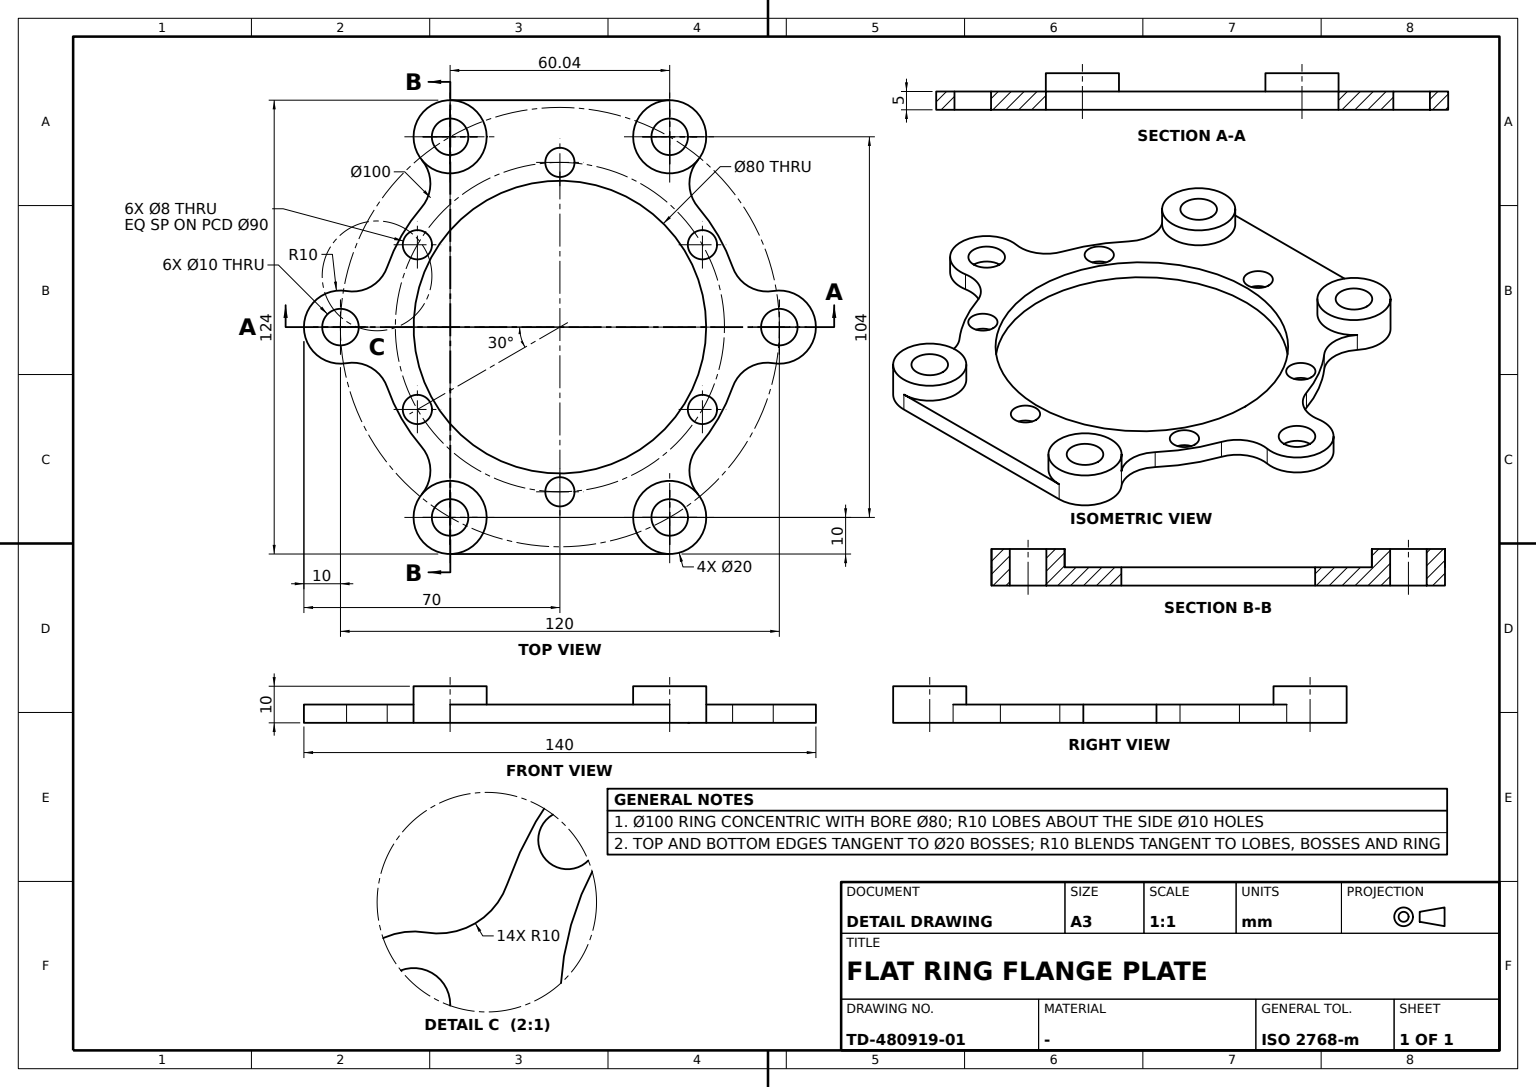
ISO-10303-21;
HEADER;
FILE_DESCRIPTION((''),'2;1');
FILE_NAME('','',(''),(''),'','','');
FILE_SCHEMA(('AUTOMOTIVE_DESIGN'));
ENDSEC;
DATA;
#1=APPLICATION_CONTEXT('');
#2=PRODUCT_CONTEXT('',#1,'mechanical');
#3=PRODUCT('','','',(#2));
#4=PRODUCT_DEFINITION_FORMATION('','',#3);
#5=PRODUCT_DEFINITION_CONTEXT('',#1,'design');
#6=PRODUCT_DEFINITION('','',#4,#5);
#7=PRODUCT_DEFINITION_SHAPE('','',#6);
#8=(LENGTH_UNIT()NAMED_UNIT(*)SI_UNIT(.MILLI.,.METRE.));
#9=(NAMED_UNIT(*)PLANE_ANGLE_UNIT()SI_UNIT($,.RADIAN.));
#10=(NAMED_UNIT(*)SI_UNIT($,.STERADIAN.)SOLID_ANGLE_UNIT());
#11=UNCERTAINTY_MEASURE_WITH_UNIT(LENGTH_MEASURE(0.005),#8,'distance_accuracy_value','');
#12=(GEOMETRIC_REPRESENTATION_CONTEXT(3)GLOBAL_UNCERTAINTY_ASSIGNED_CONTEXT((#11))GLOBAL_UNIT_ASSIGNED_CONTEXT((#8,#9,#10))REPRESENTATION_CONTEXT('',''));
#13=CARTESIAN_POINT('',(-37.8388717769,32.6836317237,0.));
#14=VERTEX_POINT('',#13);
#15=CARTESIAN_POINT('',(-37.7144300651,45.6101790342,0.));
#16=VERTEX_POINT('',#15);
#17=CARTESIAN_POINT('',(-45.4066461323,39.2203580684,0.));
#18=DIRECTION('',(0.,0.,1.));
#19=DIRECTION('',(1.,0.,0.));
#20=AXIS2_PLACEMENT_3D('',#17,#18,#19);
#21=CIRCLE('',#20,10.);
#22=EDGE_CURVE('',#14,#16,#21,.T.);
#23=ORIENTED_EDGE('',*,*,#22,.T.);
#24=CARTESIAN_POINT('',(-37.7144300651,45.6101790342,-5.));
#25=VERTEX_POINT('',#24);
#26=CARTESIAN_POINT('',(-37.7144300651,45.6101790342,-2.5));
#27=VECTOR('',#18,1000.);
#28=LINE('',#26,#27);
#29=EDGE_CURVE('',#16,#25,#28,.F.);
#30=ORIENTED_EDGE('',*,*,#29,.T.);
#31=CARTESIAN_POINT('',(-37.8388717769,32.6836317237,-5.));
#32=VERTEX_POINT('',#31);
#33=CARTESIAN_POINT('',(-45.4066461323,39.2203580684,-5.));
#34=AXIS2_PLACEMENT_3D('',#33,#18,#19);
#35=CIRCLE('',#34,10.);
#36=EDGE_CURVE('',#32,#25,#35,.T.);
#37=ORIENTED_EDGE('',*,*,#36,.F.);
#38=CARTESIAN_POINT('',(-37.8388717769,32.6836317237,-2.5));
#39=LINE('',#38,#27);
#40=EDGE_CURVE('',#14,#32,#39,.F.);
#41=ORIENTED_EDGE('',*,*,#40,.F.);
#42=EDGE_LOOP('',(#23,#30,#37,#41));
#43=FACE_BOUND('',#42,.T.);
#44=CARTESIAN_POINT('',(-45.4066461323,39.2203580684,-2.5));
#45=AXIS2_PLACEMENT_3D('',#44,#18,#19);
#46=CYLINDRICAL_SURFACE('',#45,10.);
#47=ADVANCED_FACE('',(#43),#46,.F.);
#48=CARTESIAN_POINT('',(-20.0222139979,52.,5.));
#49=VERTEX_POINT('',#48);
#50=CARTESIAN_POINT('',(-30.0222139979,52.,5.));
#51=AXIS2_PLACEMENT_3D('',#50,#18,#19);
#52=CIRCLE('',#51,10.);
#53=EDGE_CURVE('',#49,#49,#52,.T.);
#54=ORIENTED_EDGE('',*,*,#53,.T.);
#55=EDGE_LOOP('',(#54));
#56=FACE_BOUND('',#55,.T.);
#57=CARTESIAN_POINT('',(-25.0222139979,52.,5.));
#58=VERTEX_POINT('',#57);
#59=CIRCLE('',#51,5.);
#60=EDGE_CURVE('',#58,#58,#59,.T.);
#61=ORIENTED_EDGE('',*,*,#60,.F.);
#62=EDGE_LOOP('',(#61));
#63=FACE_BOUND('',#62,.T.);
#64=CARTESIAN_POINT('',(0.,0.,5.));
#65=AXIS2_PLACEMENT_3D('',#64,#18,#19);
#66=PLANE('',#65);
#67=ADVANCED_FACE('',(#56,#63),#66,.T.);
#68=CARTESIAN_POINT('',(-34.9711431703,-22.5,0.));
#69=VERTEX_POINT('',#68);
#70=CARTESIAN_POINT('',(-38.9711431703,-22.5,0.));
#71=AXIS2_PLACEMENT_3D('',#70,#18,#19);
#72=CIRCLE('',#71,4.);
#73=EDGE_CURVE('',#69,#69,#72,.T.);
#74=ORIENTED_EDGE('',*,*,#73,.T.);
#75=EDGE_LOOP('',(#74));
#76=FACE_BOUND('',#75,.T.);
#77=CARTESIAN_POINT('',(-34.9711431703,-22.5,-5.));
#78=VERTEX_POINT('',#77);
#79=CARTESIAN_POINT('',(-38.9711431703,-22.5,-5.));
#80=AXIS2_PLACEMENT_3D('',#79,#18,#19);
#81=CIRCLE('',#80,4.);
#82=EDGE_CURVE('',#78,#78,#81,.T.);
#83=ORIENTED_EDGE('',*,*,#82,.F.);
#84=EDGE_LOOP('',(#83));
#85=FACE_BOUND('',#84,.T.);
#86=CARTESIAN_POINT('',(-38.9711431703,-22.5,-2.5));
#87=AXIS2_PLACEMENT_3D('',#86,#18,#19);
#88=CYLINDRICAL_SURFACE('',#87,4.);
#89=ADVANCED_FACE('',(#76,#85),#88,.F.);
#90=CARTESIAN_POINT('',(40.0222139979,52.,5.));
#91=VERTEX_POINT('',#90);
#92=CARTESIAN_POINT('',(30.0222139979,52.,5.));
#93=AXIS2_PLACEMENT_3D('',#92,#18,#19);
#94=CIRCLE('',#93,10.);
#95=EDGE_CURVE('',#91,#91,#94,.T.);
#96=ORIENTED_EDGE('',*,*,#95,.T.);
#97=EDGE_LOOP('',(#96));
#98=FACE_BOUND('',#97,.T.);
#99=CARTESIAN_POINT('',(35.0222139979,52.,5.));
#100=VERTEX_POINT('',#99);
#101=CIRCLE('',#93,5.);
#102=EDGE_CURVE('',#100,#100,#101,.T.);
#103=ORIENTED_EDGE('',*,*,#102,.F.);
#104=EDGE_LOOP('',(#103));
#105=FACE_BOUND('',#104,.T.);
#106=ADVANCED_FACE('',(#98,#105),#66,.T.);
#107=CARTESIAN_POINT('',(30.0222139669,-62.,0.));
#108=VERTEX_POINT('',#107);
#109=CARTESIAN_POINT('',(-30.0222139979,-62.,0.));
#110=VERTEX_POINT('',#109);
#111=CARTESIAN_POINT('',(30.0222139979,-62.,0.));
#112=DIRECTION('',(-1.,0.,0.));
#113=VECTOR('',#112,1000.);
#114=LINE('',#111,#113);
#115=EDGE_CURVE('',#108,#110,#114,.T.);
#116=ORIENTED_EDGE('',*,*,#115,.T.);
#117=CARTESIAN_POINT('',(-30.0222139979,-62.,-5.));
#118=VERTEX_POINT('',#117);
#119=CARTESIAN_POINT('',(-30.0222139979,-62.,2.5));
#120=LINE('',#119,#27);
#121=EDGE_CURVE('',#110,#118,#120,.F.);
#122=ORIENTED_EDGE('',*,*,#121,.T.);
#123=CARTESIAN_POINT('',(30.0222139979,-62.,-5.));
#124=VERTEX_POINT('',#123);
#125=LINE('',#123,#113);
#126=EDGE_CURVE('',#124,#118,#125,.T.);
#127=ORIENTED_EDGE('',*,*,#126,.F.);
#128=CARTESIAN_POINT('',(30.0222139979,-62.,2.5));
#129=LINE('',#128,#27);
#130=EDGE_CURVE('',#108,#124,#129,.F.);
#131=ORIENTED_EDGE('',*,*,#130,.F.);
#132=EDGE_LOOP('',(#116,#122,#127,#131));
#133=FACE_BOUND('',#132,.T.);
#134=DIRECTION('',(0.,-1.,0.));
#135=AXIS2_PLACEMENT_3D('',#111,#134,#112);
#136=PLANE('',#135);
#137=ADVANCED_FACE('',(#133),#136,.T.);
#138=CARTESIAN_POINT('',(37.8388717769,-32.6836317237,-5.));
#139=VERTEX_POINT('',#138);
#140=CARTESIAN_POINT('',(47.2222222222,-16.4335549531,-5.));
#141=VERTEX_POINT('',#140);
#142=CARTESIAN_POINT('',(0.,0.,-5.));
#143=AXIS2_PLACEMENT_3D('',#142,#18,#19);
#144=CIRCLE('',#143,50.);
#145=EDGE_CURVE('',#139,#141,#144,.T.);
#146=ORIENTED_EDGE('',*,*,#145,.T.);
#147=CARTESIAN_POINT('',(47.2222222222,-16.4335549531,0.));
#148=VERTEX_POINT('',#147);
#149=CARTESIAN_POINT('',(47.2222222222,-16.4335549531,-2.5));
#150=LINE('',#149,#27);
#151=EDGE_CURVE('',#148,#141,#150,.F.);
#152=ORIENTED_EDGE('',*,*,#151,.F.);
#153=CARTESIAN_POINT('',(37.8388717769,-32.6836317237,0.));
#154=VERTEX_POINT('',#153);
#155=CARTESIAN_POINT('',(0.,0.,0.));
#156=AXIS2_PLACEMENT_3D('',#155,#18,#19);
#157=CIRCLE('',#156,50.);
#158=EDGE_CURVE('',#154,#148,#157,.T.);
#159=ORIENTED_EDGE('',*,*,#158,.F.);
#160=CARTESIAN_POINT('',(37.8388717769,-32.6836317237,-2.5));
#161=LINE('',#160,#27);
#162=EDGE_CURVE('',#154,#139,#161,.F.);
#163=ORIENTED_EDGE('',*,*,#162,.T.);
#164=EDGE_LOOP('',(#146,#152,#159,#163));
#165=FACE_BOUND('',#164,.T.);
#166=CARTESIAN_POINT('',(0.,0.,-2.5));
#167=AXIS2_PLACEMENT_3D('',#166,#18,#19);
#168=CYLINDRICAL_SURFACE('',#167,50.);
#169=ADVANCED_FACE('',(#165),#168,.T.);
#170=ORIENTED_EDGE('',*,*,#53,.F.);
#171=EDGE_LOOP('',(#170));
#172=FACE_BOUND('',#171,.T.);
#173=CARTESIAN_POINT('',(-30.0222139979,62.,0.));
#174=VERTEX_POINT('',#173);
#175=CARTESIAN_POINT('',(-30.0222139979,62.,-5.));
#176=VERTEX_POINT('',#175);
#177=CARTESIAN_POINT('',(-30.0222139979,62.,2.5));
#178=LINE('',#177,#27);
#179=EDGE_CURVE('',#174,#176,#178,.F.);
#180=ORIENTED_EDGE('',*,*,#179,.T.);
#181=CARTESIAN_POINT('',(-30.0222139979,52.,-5.));
#182=AXIS2_PLACEMENT_3D('',#181,#18,#19);
#183=CIRCLE('',#182,10.);
#184=EDGE_CURVE('',#176,#25,#183,.T.);
#185=ORIENTED_EDGE('',*,*,#184,.T.);
#186=ORIENTED_EDGE('',*,*,#29,.F.);
#187=CARTESIAN_POINT('',(-30.0222139979,52.,0.));
#188=AXIS2_PLACEMENT_3D('',#187,#18,#19);
#189=CIRCLE('',#188,10.);
#190=EDGE_CURVE('',#16,#174,#189,.T.);
#191=ORIENTED_EDGE('',*,*,#190,.T.);
#192=EDGE_LOOP('',(#180,#185,#186,#191));
#193=FACE_BOUND('',#192,.T.);
#194=CARTESIAN_POINT('',(-30.0222139979,52.,2.5));
#195=AXIS2_PLACEMENT_3D('',#194,#18,#19);
#196=CYLINDRICAL_SURFACE('',#195,10.);
#197=ADVANCED_FACE('',(#172,#193),#196,.T.);
#198=CARTESIAN_POINT('',(-58.3333333333,-9.8601329718,0.));
#199=VERTEX_POINT('',#198);
#200=CARTESIAN_POINT('',(-58.3333333333,-9.8601329718,-5.));
#201=VERTEX_POINT('',#200);
#202=CARTESIAN_POINT('',(-58.3333333333,-9.8601329718,-2.5));
#203=LINE('',#202,#27);
#204=EDGE_CURVE('',#199,#201,#203,.F.);
#205=ORIENTED_EDGE('',*,*,#204,.T.);
#206=CARTESIAN_POINT('',(-47.2222222222,-16.4335549531,-5.));
#207=VERTEX_POINT('',#206);
#208=CARTESIAN_POINT('',(-56.6666666667,-19.7202659437,-5.));
#209=AXIS2_PLACEMENT_3D('',#208,#18,#19);
#210=CIRCLE('',#209,10.);
#211=EDGE_CURVE('',#207,#201,#210,.T.);
#212=ORIENTED_EDGE('',*,*,#211,.F.);
#213=CARTESIAN_POINT('',(-47.2222222222,-16.4335549531,0.));
#214=VERTEX_POINT('',#213);
#215=CARTESIAN_POINT('',(-47.2222222222,-16.4335549531,-2.5));
#216=LINE('',#215,#27);
#217=EDGE_CURVE('',#214,#207,#216,.F.);
#218=ORIENTED_EDGE('',*,*,#217,.F.);
#219=CARTESIAN_POINT('',(-56.6666666667,-19.7202659437,0.));
#220=AXIS2_PLACEMENT_3D('',#219,#18,#19);
#221=CIRCLE('',#220,10.);
#222=EDGE_CURVE('',#214,#199,#221,.T.);
#223=ORIENTED_EDGE('',*,*,#222,.T.);
#224=EDGE_LOOP('',(#205,#212,#218,#223));
#225=FACE_BOUND('',#224,.T.);
#226=CARTESIAN_POINT('',(-56.6666666667,-19.7202659437,-2.5));
#227=AXIS2_PLACEMENT_3D('',#226,#18,#19);
#228=CYLINDRICAL_SURFACE('',#227,10.);
#229=ADVANCED_FACE('',(#225),#228,.F.);
#230=CARTESIAN_POINT('',(-55.,0.,-5.));
#231=VERTEX_POINT('',#230);
#232=CARTESIAN_POINT('',(-60.,0.,-5.));
#233=AXIS2_PLACEMENT_3D('',#232,#18,#19);
#234=CIRCLE('',#233,5.);
#235=EDGE_CURVE('',#231,#231,#234,.T.);
#236=ORIENTED_EDGE('',*,*,#235,.T.);
#237=EDGE_LOOP('',(#236));
#238=FACE_BOUND('',#237,.T.);
#239=CARTESIAN_POINT('',(42.9711431703,-22.5,-5.));
#240=VERTEX_POINT('',#239);
#241=CARTESIAN_POINT('',(38.9711431703,-22.5,-5.));
#242=AXIS2_PLACEMENT_3D('',#241,#18,#19);
#243=CIRCLE('',#242,4.);
#244=EDGE_CURVE('',#240,#240,#243,.T.);
#245=ORIENTED_EDGE('',*,*,#244,.T.);
#246=EDGE_LOOP('',(#245));
#247=FACE_BOUND('',#246,.T.);
#248=CARTESIAN_POINT('',(4.,45.,-5.));
#249=VERTEX_POINT('',#248);
#250=CARTESIAN_POINT('',(0.,45.,-5.));
#251=AXIS2_PLACEMENT_3D('',#250,#18,#19);
#252=CIRCLE('',#251,4.);
#253=EDGE_CURVE('',#249,#249,#252,.T.);
#254=ORIENTED_EDGE('',*,*,#253,.T.);
#255=EDGE_LOOP('',(#254));
#256=FACE_BOUND('',#255,.T.);
#257=CARTESIAN_POINT('',(-34.9711431703,22.5,-5.));
#258=VERTEX_POINT('',#257);
#259=CARTESIAN_POINT('',(-38.9711431703,22.5,-5.));
#260=AXIS2_PLACEMENT_3D('',#259,#18,#19);
#261=CIRCLE('',#260,4.);
#262=EDGE_CURVE('',#258,#258,#261,.T.);
#263=ORIENTED_EDGE('',*,*,#262,.T.);
#264=EDGE_LOOP('',(#263));
#265=FACE_BOUND('',#264,.T.);
#266=CARTESIAN_POINT('',(40.,0.,-5.));
#267=VERTEX_POINT('',#266);
#268=CIRCLE('',#143,40.);
#269=EDGE_CURVE('',#267,#267,#268,.T.);
#270=ORIENTED_EDGE('',*,*,#269,.T.);
#271=EDGE_LOOP('',(#270));
#272=FACE_BOUND('',#271,.T.);
#273=CARTESIAN_POINT('',(4.,-45.,-5.));
#274=VERTEX_POINT('',#273);
#275=CARTESIAN_POINT('',(0.,-45.,-5.));
#276=AXIS2_PLACEMENT_3D('',#275,#18,#19);
#277=CIRCLE('',#276,4.);
#278=EDGE_CURVE('',#274,#274,#277,.T.);
#279=ORIENTED_EDGE('',*,*,#278,.T.);
#280=EDGE_LOOP('',(#279));
#281=FACE_BOUND('',#280,.T.);
#282=CARTESIAN_POINT('',(-25.0222139979,52.,-5.));
#283=VERTEX_POINT('',#282);
#284=CIRCLE('',#182,5.);
#285=EDGE_CURVE('',#283,#283,#284,.T.);
#286=ORIENTED_EDGE('',*,*,#285,.T.);
#287=EDGE_LOOP('',(#286));
#288=FACE_BOUND('',#287,.T.);
#289=ORIENTED_EDGE('',*,*,#82,.T.);
#290=EDGE_LOOP('',(#289));
#291=FACE_BOUND('',#290,.T.);
#292=CARTESIAN_POINT('',(35.0222139979,52.,-5.));
#293=VERTEX_POINT('',#292);
#294=CARTESIAN_POINT('',(30.0222139979,52.,-5.));
#295=AXIS2_PLACEMENT_3D('',#294,#18,#19);
#296=CIRCLE('',#295,5.);
#297=EDGE_CURVE('',#293,#293,#296,.T.);
#298=ORIENTED_EDGE('',*,*,#297,.T.);
#299=EDGE_LOOP('',(#298));
#300=FACE_BOUND('',#299,.T.);
#301=CARTESIAN_POINT('',(-47.2222222222,16.4335549531,-5.));
#302=VERTEX_POINT('',#301);
#303=EDGE_CURVE('',#32,#302,#144,.T.);
#304=ORIENTED_EDGE('',*,*,#303,.F.);
#305=ORIENTED_EDGE('',*,*,#36,.T.);
#306=ORIENTED_EDGE('',*,*,#184,.F.);
#307=CARTESIAN_POINT('',(30.0222103757,62.,-5.));
#308=VERTEX_POINT('',#307);
#309=CARTESIAN_POINT('',(30.0222139979,62.,-5.));
#310=LINE('',#309,#113);
#311=EDGE_CURVE('',#308,#176,#310,.T.);
#312=ORIENTED_EDGE('',*,*,#311,.F.);
#313=CARTESIAN_POINT('',(37.7144300651,45.6101790342,-5.));
#314=VERTEX_POINT('',#313);
#315=CIRCLE('',#295,10.);
#316=EDGE_CURVE('',#314,#308,#315,.T.);
#317=ORIENTED_EDGE('',*,*,#316,.F.);
#318=CARTESIAN_POINT('',(37.8388717769,32.6836317237,-5.));
#319=VERTEX_POINT('',#318);
#320=CARTESIAN_POINT('',(45.4066461323,39.2203580684,-5.));
#321=AXIS2_PLACEMENT_3D('',#320,#18,#19);
#322=CIRCLE('',#321,10.);
#323=EDGE_CURVE('',#314,#319,#322,.T.);
#324=ORIENTED_EDGE('',*,*,#323,.T.);
#325=CARTESIAN_POINT('',(47.2222222222,16.4335549531,-5.));
#326=VERTEX_POINT('',#325);
#327=EDGE_CURVE('',#326,#319,#144,.T.);
#328=ORIENTED_EDGE('',*,*,#327,.F.);
#329=CARTESIAN_POINT('',(58.3333333333,9.8601329718,-5.));
#330=VERTEX_POINT('',#329);
#331=CARTESIAN_POINT('',(56.6666666667,19.7202659437,-5.));
#332=AXIS2_PLACEMENT_3D('',#331,#18,#19);
#333=CIRCLE('',#332,10.);
#334=EDGE_CURVE('',#326,#330,#333,.T.);
#335=ORIENTED_EDGE('',*,*,#334,.T.);
#336=CARTESIAN_POINT('',(58.3333333333,-9.8601329718,-5.));
#337=VERTEX_POINT('',#336);
#338=CARTESIAN_POINT('',(60.,0.,-5.));
#339=AXIS2_PLACEMENT_3D('',#338,#18,#19);
#340=CIRCLE('',#339,10.);
#341=EDGE_CURVE('',#337,#330,#340,.T.);
#342=ORIENTED_EDGE('',*,*,#341,.F.);
#343=CARTESIAN_POINT('',(56.6666666667,-19.7202659437,-5.));
#344=AXIS2_PLACEMENT_3D('',#343,#18,#19);
#345=CIRCLE('',#344,10.);
#346=EDGE_CURVE('',#337,#141,#345,.T.);
#347=ORIENTED_EDGE('',*,*,#346,.T.);
#348=ORIENTED_EDGE('',*,*,#145,.F.);
#349=CARTESIAN_POINT('',(37.7144300651,-45.6101790342,-5.));
#350=VERTEX_POINT('',#349);
#351=CARTESIAN_POINT('',(45.4066461323,-39.2203580684,-5.));
#352=AXIS2_PLACEMENT_3D('',#351,#18,#19);
#353=CIRCLE('',#352,10.);
#354=EDGE_CURVE('',#139,#350,#353,.T.);
#355=ORIENTED_EDGE('',*,*,#354,.T.);
#356=CARTESIAN_POINT('',(30.0222139979,-52.,-5.));
#357=AXIS2_PLACEMENT_3D('',#356,#18,#19);
#358=CIRCLE('',#357,10.);
#359=EDGE_CURVE('',#124,#350,#358,.T.);
#360=ORIENTED_EDGE('',*,*,#359,.F.);
#361=ORIENTED_EDGE('',*,*,#126,.T.);
#362=CARTESIAN_POINT('',(-37.7144300651,-45.6101790342,-5.));
#363=VERTEX_POINT('',#362);
#364=CARTESIAN_POINT('',(-30.0222139979,-52.,-5.));
#365=AXIS2_PLACEMENT_3D('',#364,#18,#19);
#366=CIRCLE('',#365,10.);
#367=EDGE_CURVE('',#363,#118,#366,.T.);
#368=ORIENTED_EDGE('',*,*,#367,.F.);
#369=CARTESIAN_POINT('',(-37.8388717769,-32.6836317237,-5.));
#370=VERTEX_POINT('',#369);
#371=CARTESIAN_POINT('',(-45.4066461323,-39.2203580684,-5.));
#372=AXIS2_PLACEMENT_3D('',#371,#18,#19);
#373=CIRCLE('',#372,10.);
#374=EDGE_CURVE('',#363,#370,#373,.T.);
#375=ORIENTED_EDGE('',*,*,#374,.T.);
#376=EDGE_CURVE('',#207,#370,#144,.T.);
#377=ORIENTED_EDGE('',*,*,#376,.F.);
#378=ORIENTED_EDGE('',*,*,#211,.T.);
#379=CARTESIAN_POINT('',(-58.3333333333,9.8601329718,-5.));
#380=VERTEX_POINT('',#379);
#381=CIRCLE('',#233,10.);
#382=EDGE_CURVE('',#380,#201,#381,.T.);
#383=ORIENTED_EDGE('',*,*,#382,.F.);
#384=CARTESIAN_POINT('',(-56.6666666667,19.7202659437,-5.));
#385=AXIS2_PLACEMENT_3D('',#384,#18,#19);
#386=CIRCLE('',#385,10.);
#387=EDGE_CURVE('',#380,#302,#386,.T.);
#388=ORIENTED_EDGE('',*,*,#387,.T.);
#389=EDGE_LOOP('',(#304,#305,#306,#312,#317,#324,#328,#335,#342,#347,#348,#355,#360,#361,#368,#375,#377,#378,#383,#388));
#390=FACE_BOUND('',#389,.T.);
#391=CARTESIAN_POINT('',(-25.0222139979,-52.,-5.));
#392=VERTEX_POINT('',#391);
#393=CIRCLE('',#365,5.);
#394=EDGE_CURVE('',#392,#392,#393,.T.);
#395=ORIENTED_EDGE('',*,*,#394,.T.);
#396=EDGE_LOOP('',(#395));
#397=FACE_BOUND('',#396,.T.);
#398=CARTESIAN_POINT('',(42.9711431703,22.5,-5.));
#399=VERTEX_POINT('',#398);
#400=CARTESIAN_POINT('',(38.9711431703,22.5,-5.));
#401=AXIS2_PLACEMENT_3D('',#400,#18,#19);
#402=CIRCLE('',#401,4.);
#403=EDGE_CURVE('',#399,#399,#402,.T.);
#404=ORIENTED_EDGE('',*,*,#403,.T.);
#405=EDGE_LOOP('',(#404));
#406=FACE_BOUND('',#405,.T.);
#407=CARTESIAN_POINT('',(65.,0.,-5.));
#408=VERTEX_POINT('',#407);
#409=CIRCLE('',#339,5.);
#410=EDGE_CURVE('',#408,#408,#409,.T.);
#411=ORIENTED_EDGE('',*,*,#410,.T.);
#412=EDGE_LOOP('',(#411));
#413=FACE_BOUND('',#412,.T.);
#414=CARTESIAN_POINT('',(35.0222139979,-52.,-5.));
#415=VERTEX_POINT('',#414);
#416=CIRCLE('',#357,5.);
#417=EDGE_CURVE('',#415,#415,#416,.T.);
#418=ORIENTED_EDGE('',*,*,#417,.T.);
#419=EDGE_LOOP('',(#418));
#420=FACE_BOUND('',#419,.T.);
#421=PLANE('',#143);
#422=ADVANCED_FACE('',(#238,#247,#256,#265,#272,#281,#288,#291,#300,#390,#397,#406,#413,#420),#421,.F.);
#423=ORIENTED_EDGE('',*,*,#297,.F.);
#424=EDGE_LOOP('',(#423));
#425=FACE_BOUND('',#424,.T.);
#426=ORIENTED_EDGE('',*,*,#102,.T.);
#427=EDGE_LOOP('',(#426));
#428=FACE_BOUND('',#427,.T.);
#429=CARTESIAN_POINT('',(30.0222139979,52.,2.5));
#430=AXIS2_PLACEMENT_3D('',#429,#18,#19);
#431=CYLINDRICAL_SURFACE('',#430,5.);
#432=ADVANCED_FACE('',(#425,#428),#431,.F.);
#433=ORIENTED_EDGE('',*,*,#179,.F.);
#434=CARTESIAN_POINT('',(30.0222139669,62.,0.));
#435=VERTEX_POINT('',#434);
#436=CARTESIAN_POINT('',(30.0222139979,62.,0.));
#437=LINE('',#436,#113);
#438=EDGE_CURVE('',#435,#174,#437,.T.);
#439=ORIENTED_EDGE('',*,*,#438,.F.);
#440=CARTESIAN_POINT('',(30.0222139979,62.,2.5));
#441=LINE('',#440,#27);
#442=EDGE_CURVE('',#435,#308,#441,.F.);
#443=ORIENTED_EDGE('',*,*,#442,.T.);
#444=ORIENTED_EDGE('',*,*,#311,.T.);
#445=EDGE_LOOP('',(#433,#439,#443,#444));
#446=FACE_BOUND('',#445,.T.);
#447=AXIS2_PLACEMENT_3D('',#436,#134,#112);
#448=PLANE('',#447);
#449=ADVANCED_FACE('',(#446),#448,.F.);
#450=ORIENTED_EDGE('',*,*,#417,.F.);
#451=EDGE_LOOP('',(#450));
#452=FACE_BOUND('',#451,.T.);
#453=CARTESIAN_POINT('',(35.0222139979,-52.,5.));
#454=VERTEX_POINT('',#453);
#455=CARTESIAN_POINT('',(30.0222139979,-52.,5.));
#456=AXIS2_PLACEMENT_3D('',#455,#18,#19);
#457=CIRCLE('',#456,5.);
#458=EDGE_CURVE('',#454,#454,#457,.T.);
#459=ORIENTED_EDGE('',*,*,#458,.T.);
#460=EDGE_LOOP('',(#459));
#461=FACE_BOUND('',#460,.T.);
#462=CARTESIAN_POINT('',(30.0222139979,-52.,2.5));
#463=AXIS2_PLACEMENT_3D('',#462,#18,#19);
#464=CYLINDRICAL_SURFACE('',#463,5.);
#465=ADVANCED_FACE('',(#452,#461),#464,.F.);
#466=ORIENTED_EDGE('',*,*,#359,.T.);
#467=CARTESIAN_POINT('',(37.7144300651,-45.6101790342,0.));
#468=VERTEX_POINT('',#467);
#469=CARTESIAN_POINT('',(37.7144300651,-45.6101790342,-2.4999999792));
#470=LINE('',#469,#27);
#471=EDGE_CURVE('',#468,#350,#470,.F.);
#472=ORIENTED_EDGE('',*,*,#471,.F.);
#473=CARTESIAN_POINT('',(30.0222139979,-52.,0.));
#474=AXIS2_PLACEMENT_3D('',#473,#18,#19);
#475=CIRCLE('',#474,10.);
#476=EDGE_CURVE('',#468,#108,#475,.T.);
#477=ORIENTED_EDGE('',*,*,#476,.T.);
#478=ORIENTED_EDGE('',*,*,#130,.T.);
#479=EDGE_LOOP('',(#466,#472,#477,#478));
#480=FACE_BOUND('',#479,.T.);
#481=CARTESIAN_POINT('',(40.0222139979,-52.,5.));
#482=VERTEX_POINT('',#481);
#483=CIRCLE('',#456,10.);
#484=EDGE_CURVE('',#482,#482,#483,.T.);
#485=ORIENTED_EDGE('',*,*,#484,.F.);
#486=EDGE_LOOP('',(#485));
#487=FACE_BOUND('',#486,.T.);
#488=CYLINDRICAL_SURFACE('',#463,10.);
#489=ADVANCED_FACE('',(#480,#487),#488,.T.);
#490=CARTESIAN_POINT('',(-47.2222222222,16.4335549531,0.));
#491=VERTEX_POINT('',#490);
#492=CARTESIAN_POINT('',(-47.2222222222,16.4335549531,-2.5));
#493=LINE('',#492,#27);
#494=EDGE_CURVE('',#491,#302,#493,.F.);
#495=ORIENTED_EDGE('',*,*,#494,.F.);
#496=EDGE_CURVE('',#14,#491,#157,.T.);
#497=ORIENTED_EDGE('',*,*,#496,.F.);
#498=ORIENTED_EDGE('',*,*,#40,.T.);
#499=ORIENTED_EDGE('',*,*,#303,.T.);
#500=EDGE_LOOP('',(#495,#497,#498,#499));
#501=FACE_BOUND('',#500,.T.);
#502=ADVANCED_FACE('',(#501),#168,.T.);
#503=CARTESIAN_POINT('',(58.3333333333,-9.8601329718,0.));
#504=VERTEX_POINT('',#503);
#505=CARTESIAN_POINT('',(58.3333333333,9.8601329718,0.));
#506=VERTEX_POINT('',#505);
#507=CARTESIAN_POINT('',(60.,0.,0.));
#508=AXIS2_PLACEMENT_3D('',#507,#18,#19);
#509=CIRCLE('',#508,10.);
#510=EDGE_CURVE('',#504,#506,#509,.T.);
#511=ORIENTED_EDGE('',*,*,#510,.F.);
#512=CARTESIAN_POINT('',(58.3333333333,-9.8601329718,-2.5));
#513=LINE('',#512,#27);
#514=EDGE_CURVE('',#504,#337,#513,.F.);
#515=ORIENTED_EDGE('',*,*,#514,.T.);
#516=ORIENTED_EDGE('',*,*,#341,.T.);
#517=CARTESIAN_POINT('',(58.3333333333,9.8601329718,-2.5));
#518=LINE('',#517,#27);
#519=EDGE_CURVE('',#506,#330,#518,.F.);
#520=ORIENTED_EDGE('',*,*,#519,.F.);
#521=EDGE_LOOP('',(#511,#515,#516,#520));
#522=FACE_BOUND('',#521,.T.);
#523=CARTESIAN_POINT('',(60.,0.,-2.5));
#524=AXIS2_PLACEMENT_3D('',#523,#18,#19);
#525=CYLINDRICAL_SURFACE('',#524,10.);
#526=ADVANCED_FACE('',(#522),#525,.T.);
#527=CARTESIAN_POINT('',(-58.3333333333,9.8601329718,0.));
#528=VERTEX_POINT('',#527);
#529=CARTESIAN_POINT('',(-56.6666666667,19.7202659437,0.));
#530=AXIS2_PLACEMENT_3D('',#529,#18,#19);
#531=CIRCLE('',#530,10.);
#532=EDGE_CURVE('',#528,#491,#531,.T.);
#533=ORIENTED_EDGE('',*,*,#532,.T.);
#534=ORIENTED_EDGE('',*,*,#494,.T.);
#535=ORIENTED_EDGE('',*,*,#387,.F.);
#536=CARTESIAN_POINT('',(-58.3333333333,9.8601329718,-2.5));
#537=LINE('',#536,#27);
#538=EDGE_CURVE('',#528,#380,#537,.F.);
#539=ORIENTED_EDGE('',*,*,#538,.F.);
#540=EDGE_LOOP('',(#533,#534,#535,#539));
#541=FACE_BOUND('',#540,.T.);
#542=CARTESIAN_POINT('',(-56.6666666667,19.7202659437,-2.5));
#543=AXIS2_PLACEMENT_3D('',#542,#18,#19);
#544=CYLINDRICAL_SURFACE('',#543,10.);
#545=ADVANCED_FACE('',(#541),#544,.F.);
#546=ORIENTED_EDGE('',*,*,#471,.T.);
#547=ORIENTED_EDGE('',*,*,#354,.F.);
#548=ORIENTED_EDGE('',*,*,#162,.F.);
#549=CARTESIAN_POINT('',(45.4066461323,-39.2203580684,0.));
#550=AXIS2_PLACEMENT_3D('',#549,#18,#19);
#551=CIRCLE('',#550,10.);
#552=EDGE_CURVE('',#154,#468,#551,.T.);
#553=ORIENTED_EDGE('',*,*,#552,.T.);
#554=EDGE_LOOP('',(#546,#547,#548,#553));
#555=FACE_BOUND('',#554,.T.);
#556=CARTESIAN_POINT('',(45.4066461323,-39.2203580684,-2.5));
#557=AXIS2_PLACEMENT_3D('',#556,#18,#19);
#558=CYLINDRICAL_SURFACE('',#557,10.);
#559=ADVANCED_FACE('',(#555),#558,.F.);
#560=CARTESIAN_POINT('',(-25.0222139979,-52.,5.));
#561=VERTEX_POINT('',#560);
#562=CARTESIAN_POINT('',(-30.0222139979,-52.,5.));
#563=AXIS2_PLACEMENT_3D('',#562,#18,#19);
#564=CIRCLE('',#563,5.);
#565=EDGE_CURVE('',#561,#561,#564,.T.);
#566=ORIENTED_EDGE('',*,*,#565,.F.);
#567=EDGE_LOOP('',(#566));
#568=FACE_BOUND('',#567,.T.);
#569=CARTESIAN_POINT('',(-20.0222139979,-52.,5.));
#570=VERTEX_POINT('',#569);
#571=CIRCLE('',#563,10.);
#572=EDGE_CURVE('',#570,#570,#571,.T.);
#573=ORIENTED_EDGE('',*,*,#572,.T.);
#574=EDGE_LOOP('',(#573));
#575=FACE_BOUND('',#574,.T.);
#576=ADVANCED_FACE('',(#568,#575),#66,.T.);
#577=CARTESIAN_POINT('',(42.9711431703,-22.5,0.));
#578=VERTEX_POINT('',#577);
#579=CARTESIAN_POINT('',(38.9711431703,-22.5,0.));
#580=AXIS2_PLACEMENT_3D('',#579,#18,#19);
#581=CIRCLE('',#580,4.);
#582=EDGE_CURVE('',#578,#578,#581,.T.);
#583=ORIENTED_EDGE('',*,*,#582,.T.);
#584=EDGE_LOOP('',(#583));
#585=FACE_BOUND('',#584,.T.);
#586=ORIENTED_EDGE('',*,*,#244,.F.);
#587=EDGE_LOOP('',(#586));
#588=FACE_BOUND('',#587,.T.);
#589=CARTESIAN_POINT('',(38.9711431703,-22.5,-2.5));
#590=AXIS2_PLACEMENT_3D('',#589,#18,#19);
#591=CYLINDRICAL_SURFACE('',#590,4.);
#592=ADVANCED_FACE('',(#585,#588),#591,.F.);
#593=CARTESIAN_POINT('',(-37.7144300651,-45.6101790342,0.));
#594=VERTEX_POINT('',#593);
#595=CARTESIAN_POINT('',(-37.8388717769,-32.6836317237,0.));
#596=VERTEX_POINT('',#595);
#597=CARTESIAN_POINT('',(-45.4066461323,-39.2203580684,0.));
#598=AXIS2_PLACEMENT_3D('',#597,#18,#19);
#599=CIRCLE('',#598,10.);
#600=EDGE_CURVE('',#594,#596,#599,.T.);
#601=ORIENTED_EDGE('',*,*,#600,.T.);
#602=CARTESIAN_POINT('',(-37.8388717769,-32.6836317237,-2.5));
#603=LINE('',#602,#27);
#604=EDGE_CURVE('',#596,#370,#603,.F.);
#605=ORIENTED_EDGE('',*,*,#604,.T.);
#606=ORIENTED_EDGE('',*,*,#374,.F.);
#607=CARTESIAN_POINT('',(-37.7144300651,-45.6101790342,-2.5));
#608=LINE('',#607,#27);
#609=EDGE_CURVE('',#594,#363,#608,.F.);
#610=ORIENTED_EDGE('',*,*,#609,.F.);
#611=EDGE_LOOP('',(#601,#605,#606,#610));
#612=FACE_BOUND('',#611,.T.);
#613=CARTESIAN_POINT('',(-45.4066461323,-39.2203580684,-2.5));
#614=AXIS2_PLACEMENT_3D('',#613,#18,#19);
#615=CYLINDRICAL_SURFACE('',#614,10.);
#616=ADVANCED_FACE('',(#612),#615,.F.);
#617=CARTESIAN_POINT('',(37.8388717769,32.6836317237,0.));
#618=VERTEX_POINT('',#617);
#619=CARTESIAN_POINT('',(37.8388717769,32.6836317237,-2.5));
#620=LINE('',#619,#27);
#621=EDGE_CURVE('',#618,#319,#620,.F.);
#622=ORIENTED_EDGE('',*,*,#621,.F.);
#623=CARTESIAN_POINT('',(47.2222222222,16.4335549531,0.));
#624=VERTEX_POINT('',#623);
#625=EDGE_CURVE('',#624,#618,#157,.T.);
#626=ORIENTED_EDGE('',*,*,#625,.F.);
#627=CARTESIAN_POINT('',(47.2222222222,16.4335549531,-2.5));
#628=LINE('',#627,#27);
#629=EDGE_CURVE('',#624,#326,#628,.F.);
#630=ORIENTED_EDGE('',*,*,#629,.T.);
#631=ORIENTED_EDGE('',*,*,#327,.T.);
#632=EDGE_LOOP('',(#622,#626,#630,#631));
#633=FACE_BOUND('',#632,.T.);
#634=ADVANCED_FACE('',(#633),#168,.T.);
#635=ORIENTED_EDGE('',*,*,#403,.F.);
#636=EDGE_LOOP('',(#635));
#637=FACE_BOUND('',#636,.T.);
#638=CARTESIAN_POINT('',(42.9711431703,22.5,0.));
#639=VERTEX_POINT('',#638);
#640=CARTESIAN_POINT('',(38.9711431703,22.5,0.));
#641=AXIS2_PLACEMENT_3D('',#640,#18,#19);
#642=CIRCLE('',#641,4.);
#643=EDGE_CURVE('',#639,#639,#642,.T.);
#644=ORIENTED_EDGE('',*,*,#643,.T.);
#645=EDGE_LOOP('',(#644));
#646=FACE_BOUND('',#645,.T.);
#647=CARTESIAN_POINT('',(38.9711431703,22.5,-2.5));
#648=AXIS2_PLACEMENT_3D('',#647,#18,#19);
#649=CYLINDRICAL_SURFACE('',#648,4.);
#650=ADVANCED_FACE('',(#637,#646),#649,.F.);
#651=ORIENTED_EDGE('',*,*,#565,.T.);
#652=EDGE_LOOP('',(#651));
#653=FACE_BOUND('',#652,.T.);
#654=ORIENTED_EDGE('',*,*,#394,.F.);
#655=EDGE_LOOP('',(#654));
#656=FACE_BOUND('',#655,.T.);
#657=CARTESIAN_POINT('',(-30.0222139979,-52.,2.5));
#658=AXIS2_PLACEMENT_3D('',#657,#18,#19);
#659=CYLINDRICAL_SURFACE('',#658,5.);
#660=ADVANCED_FACE('',(#653,#656),#659,.F.);
#661=CARTESIAN_POINT('',(-34.9711431703,22.5,0.));
#662=VERTEX_POINT('',#661);
#663=CARTESIAN_POINT('',(-38.9711431703,22.5,0.));
#664=AXIS2_PLACEMENT_3D('',#663,#18,#19);
#665=CIRCLE('',#664,4.);
#666=EDGE_CURVE('',#662,#662,#665,.T.);
#667=ORIENTED_EDGE('',*,*,#666,.T.);
#668=EDGE_LOOP('',(#667));
#669=FACE_BOUND('',#668,.T.);
#670=ORIENTED_EDGE('',*,*,#262,.F.);
#671=EDGE_LOOP('',(#670));
#672=FACE_BOUND('',#671,.T.);
#673=CARTESIAN_POINT('',(-38.9711431703,22.5,-2.5));
#674=AXIS2_PLACEMENT_3D('',#673,#18,#19);
#675=CYLINDRICAL_SURFACE('',#674,4.);
#676=ADVANCED_FACE('',(#669,#672),#675,.F.);
#677=ORIENTED_EDGE('',*,*,#410,.F.);
#678=EDGE_LOOP('',(#677));
#679=FACE_BOUND('',#678,.T.);
#680=CARTESIAN_POINT('',(65.,0.,0.));
#681=VERTEX_POINT('',#680);
#682=CIRCLE('',#508,5.);
#683=EDGE_CURVE('',#681,#681,#682,.T.);
#684=ORIENTED_EDGE('',*,*,#683,.T.);
#685=EDGE_LOOP('',(#684));
#686=FACE_BOUND('',#685,.T.);
#687=CYLINDRICAL_SURFACE('',#524,5.);
#688=ADVANCED_FACE('',(#679,#686),#687,.F.);
#689=CARTESIAN_POINT('',(4.,-45.,0.));
#690=VERTEX_POINT('',#689);
#691=CARTESIAN_POINT('',(0.,-45.,0.));
#692=AXIS2_PLACEMENT_3D('',#691,#18,#19);
#693=CIRCLE('',#692,4.);
#694=EDGE_CURVE('',#690,#690,#693,.T.);
#695=ORIENTED_EDGE('',*,*,#694,.F.);
#696=EDGE_LOOP('',(#695));
#697=FACE_BOUND('',#696,.T.);
#698=CARTESIAN_POINT('',(4.,45.,0.));
#699=VERTEX_POINT('',#698);
#700=CARTESIAN_POINT('',(0.,45.,0.));
#701=AXIS2_PLACEMENT_3D('',#700,#18,#19);
#702=CIRCLE('',#701,4.);
#703=EDGE_CURVE('',#699,#699,#702,.T.);
#704=ORIENTED_EDGE('',*,*,#703,.F.);
#705=EDGE_LOOP('',(#704));
#706=FACE_BOUND('',#705,.T.);
#707=ORIENTED_EDGE('',*,*,#643,.F.);
#708=EDGE_LOOP('',(#707));
#709=FACE_BOUND('',#708,.T.);
#710=CARTESIAN_POINT('',(40.,0.,0.));
#711=VERTEX_POINT('',#710);
#712=CIRCLE('',#156,40.);
#713=EDGE_CURVE('',#711,#711,#712,.T.);
#714=ORIENTED_EDGE('',*,*,#713,.F.);
#715=EDGE_LOOP('',(#714));
#716=FACE_BOUND('',#715,.T.);
#717=ORIENTED_EDGE('',*,*,#582,.F.);
#718=EDGE_LOOP('',(#717));
#719=FACE_BOUND('',#718,.T.);
#720=ORIENTED_EDGE('',*,*,#666,.F.);
#721=EDGE_LOOP('',(#720));
#722=FACE_BOUND('',#721,.T.);
#723=ORIENTED_EDGE('',*,*,#73,.F.);
#724=EDGE_LOOP('',(#723));
#725=FACE_BOUND('',#724,.T.);
#726=ORIENTED_EDGE('',*,*,#158,.T.);
#727=CARTESIAN_POINT('',(56.6666666667,-19.7202659437,0.));
#728=AXIS2_PLACEMENT_3D('',#727,#18,#19);
#729=CIRCLE('',#728,10.);
#730=EDGE_CURVE('',#504,#148,#729,.T.);
#731=ORIENTED_EDGE('',*,*,#730,.F.);
#732=ORIENTED_EDGE('',*,*,#510,.T.);
#733=CARTESIAN_POINT('',(56.6666666667,19.7202659437,0.));
#734=AXIS2_PLACEMENT_3D('',#733,#18,#19);
#735=CIRCLE('',#734,10.);
#736=EDGE_CURVE('',#624,#506,#735,.T.);
#737=ORIENTED_EDGE('',*,*,#736,.F.);
#738=ORIENTED_EDGE('',*,*,#625,.T.);
#739=CARTESIAN_POINT('',(37.7144300651,45.6101790342,0.));
#740=VERTEX_POINT('',#739);
#741=CARTESIAN_POINT('',(45.4066461323,39.2203580684,0.));
#742=AXIS2_PLACEMENT_3D('',#741,#18,#19);
#743=CIRCLE('',#742,10.);
#744=EDGE_CURVE('',#740,#618,#743,.T.);
#745=ORIENTED_EDGE('',*,*,#744,.F.);
#746=CARTESIAN_POINT('',(30.0222139979,52.,0.));
#747=AXIS2_PLACEMENT_3D('',#746,#18,#19);
#748=CIRCLE('',#747,10.);
#749=EDGE_CURVE('',#435,#740,#748,.T.);
#750=ORIENTED_EDGE('',*,*,#749,.F.);
#751=ORIENTED_EDGE('',*,*,#438,.T.);
#752=ORIENTED_EDGE('',*,*,#190,.F.);
#753=ORIENTED_EDGE('',*,*,#22,.F.);
#754=ORIENTED_EDGE('',*,*,#496,.T.);
#755=ORIENTED_EDGE('',*,*,#532,.F.);
#756=CARTESIAN_POINT('',(-60.,0.,0.));
#757=AXIS2_PLACEMENT_3D('',#756,#18,#19);
#758=CIRCLE('',#757,10.);
#759=EDGE_CURVE('',#528,#199,#758,.T.);
#760=ORIENTED_EDGE('',*,*,#759,.T.);
#761=ORIENTED_EDGE('',*,*,#222,.F.);
#762=EDGE_CURVE('',#214,#596,#157,.T.);
#763=ORIENTED_EDGE('',*,*,#762,.T.);
#764=ORIENTED_EDGE('',*,*,#600,.F.);
#765=CARTESIAN_POINT('',(-30.0222139979,-52.,0.));
#766=AXIS2_PLACEMENT_3D('',#765,#18,#19);
#767=CIRCLE('',#766,10.);
#768=EDGE_CURVE('',#110,#594,#767,.T.);
#769=ORIENTED_EDGE('',*,*,#768,.F.);
#770=ORIENTED_EDGE('',*,*,#115,.F.);
#771=ORIENTED_EDGE('',*,*,#476,.F.);
#772=ORIENTED_EDGE('',*,*,#552,.F.);
#773=EDGE_LOOP('',(#726,#731,#732,#737,#738,#745,#750,#751,#752,#753,#754,#755,#760,#761,#763,#764,#769,#770,#771,#772));
#774=FACE_BOUND('',#773,.T.);
#775=ORIENTED_EDGE('',*,*,#683,.F.);
#776=EDGE_LOOP('',(#775));
#777=FACE_BOUND('',#776,.T.);
#778=CARTESIAN_POINT('',(-55.,0.,0.));
#779=VERTEX_POINT('',#778);
#780=CIRCLE('',#757,5.);
#781=EDGE_CURVE('',#779,#779,#780,.T.);
#782=ORIENTED_EDGE('',*,*,#781,.F.);
#783=EDGE_LOOP('',(#782));
#784=FACE_BOUND('',#783,.T.);
#785=PLANE('',#156);
#786=ADVANCED_FACE('',(#697,#706,#709,#716,#719,#722,#725,#774,#777,#784),#785,.T.);
#787=ORIENTED_EDGE('',*,*,#629,.F.);
#788=ORIENTED_EDGE('',*,*,#736,.T.);
#789=ORIENTED_EDGE('',*,*,#519,.T.);
#790=ORIENTED_EDGE('',*,*,#334,.F.);
#791=EDGE_LOOP('',(#787,#788,#789,#790));
#792=FACE_BOUND('',#791,.T.);
#793=CARTESIAN_POINT('',(56.6666666667,19.7202659437,-2.5));
#794=AXIS2_PLACEMENT_3D('',#793,#18,#19);
#795=CYLINDRICAL_SURFACE('',#794,10.);
#796=ADVANCED_FACE('',(#792),#795,.F.);
#797=ORIENTED_EDGE('',*,*,#781,.T.);
#798=EDGE_LOOP('',(#797));
#799=FACE_BOUND('',#798,.T.);
#800=ORIENTED_EDGE('',*,*,#235,.F.);
#801=EDGE_LOOP('',(#800));
#802=FACE_BOUND('',#801,.T.);
#803=CARTESIAN_POINT('',(-60.,0.,-2.5));
#804=AXIS2_PLACEMENT_3D('',#803,#18,#19);
#805=CYLINDRICAL_SURFACE('',#804,5.);
#806=ADVANCED_FACE('',(#799,#802),#805,.F.);
#807=ORIENTED_EDGE('',*,*,#730,.T.);
#808=ORIENTED_EDGE('',*,*,#151,.T.);
#809=ORIENTED_EDGE('',*,*,#346,.F.);
#810=ORIENTED_EDGE('',*,*,#514,.F.);
#811=EDGE_LOOP('',(#807,#808,#809,#810));
#812=FACE_BOUND('',#811,.T.);
#813=CARTESIAN_POINT('',(56.6666666667,-19.7202659437,-2.5));
#814=AXIS2_PLACEMENT_3D('',#813,#18,#19);
#815=CYLINDRICAL_SURFACE('',#814,10.);
#816=ADVANCED_FACE('',(#812),#815,.F.);
#817=ORIENTED_EDGE('',*,*,#609,.T.);
#818=ORIENTED_EDGE('',*,*,#367,.T.);
#819=ORIENTED_EDGE('',*,*,#121,.F.);
#820=ORIENTED_EDGE('',*,*,#768,.T.);
#821=EDGE_LOOP('',(#817,#818,#819,#820));
#822=FACE_BOUND('',#821,.T.);
#823=ORIENTED_EDGE('',*,*,#572,.F.);
#824=EDGE_LOOP('',(#823));
#825=FACE_BOUND('',#824,.T.);
#826=CYLINDRICAL_SURFACE('',#658,10.);
#827=ADVANCED_FACE('',(#822,#825),#826,.T.);
#828=ORIENTED_EDGE('',*,*,#538,.T.);
#829=ORIENTED_EDGE('',*,*,#382,.T.);
#830=ORIENTED_EDGE('',*,*,#204,.F.);
#831=ORIENTED_EDGE('',*,*,#759,.F.);
#832=EDGE_LOOP('',(#828,#829,#830,#831));
#833=FACE_BOUND('',#832,.T.);
#834=CYLINDRICAL_SURFACE('',#804,10.);
#835=ADVANCED_FACE('',(#833),#834,.T.);
#836=ORIENTED_EDGE('',*,*,#703,.T.);
#837=EDGE_LOOP('',(#836));
#838=FACE_BOUND('',#837,.T.);
#839=ORIENTED_EDGE('',*,*,#253,.F.);
#840=EDGE_LOOP('',(#839));
#841=FACE_BOUND('',#840,.T.);
#842=CARTESIAN_POINT('',(0.,45.,-2.5));
#843=AXIS2_PLACEMENT_3D('',#842,#18,#19);
#844=CYLINDRICAL_SURFACE('',#843,4.);
#845=ADVANCED_FACE('',(#838,#841),#844,.F.);
#846=ORIENTED_EDGE('',*,*,#285,.F.);
#847=EDGE_LOOP('',(#846));
#848=FACE_BOUND('',#847,.T.);
#849=ORIENTED_EDGE('',*,*,#60,.T.);
#850=EDGE_LOOP('',(#849));
#851=FACE_BOUND('',#850,.T.);
#852=CYLINDRICAL_SURFACE('',#195,5.);
#853=ADVANCED_FACE('',(#848,#851),#852,.F.);
#854=ORIENTED_EDGE('',*,*,#278,.F.);
#855=EDGE_LOOP('',(#854));
#856=FACE_BOUND('',#855,.T.);
#857=ORIENTED_EDGE('',*,*,#694,.T.);
#858=EDGE_LOOP('',(#857));
#859=FACE_BOUND('',#858,.T.);
#860=CARTESIAN_POINT('',(0.,-45.,-2.5));
#861=AXIS2_PLACEMENT_3D('',#860,#18,#19);
#862=CYLINDRICAL_SURFACE('',#861,4.);
#863=ADVANCED_FACE('',(#856,#859),#862,.F.);
#864=ORIENTED_EDGE('',*,*,#323,.F.);
#865=CARTESIAN_POINT('',(37.7144300651,45.6101790342,-2.4999999792));
#866=LINE('',#865,#27);
#867=EDGE_CURVE('',#740,#314,#866,.F.);
#868=ORIENTED_EDGE('',*,*,#867,.F.);
#869=ORIENTED_EDGE('',*,*,#744,.T.);
#870=ORIENTED_EDGE('',*,*,#621,.T.);
#871=EDGE_LOOP('',(#864,#868,#869,#870));
#872=FACE_BOUND('',#871,.T.);
#873=CARTESIAN_POINT('',(45.4066461323,39.2203580684,-2.5));
#874=AXIS2_PLACEMENT_3D('',#873,#18,#19);
#875=CYLINDRICAL_SURFACE('',#874,10.);
#876=ADVANCED_FACE('',(#872),#875,.F.);
#877=ORIENTED_EDGE('',*,*,#604,.F.);
#878=ORIENTED_EDGE('',*,*,#762,.F.);
#879=ORIENTED_EDGE('',*,*,#217,.T.);
#880=ORIENTED_EDGE('',*,*,#376,.T.);
#881=EDGE_LOOP('',(#877,#878,#879,#880));
#882=FACE_BOUND('',#881,.T.);
#883=ADVANCED_FACE('',(#882),#168,.T.);
#884=ORIENTED_EDGE('',*,*,#458,.F.);
#885=EDGE_LOOP('',(#884));
#886=FACE_BOUND('',#885,.T.);
#887=ORIENTED_EDGE('',*,*,#484,.T.);
#888=EDGE_LOOP('',(#887));
#889=FACE_BOUND('',#888,.T.);
#890=ADVANCED_FACE('',(#886,#889),#66,.T.);
#891=ORIENTED_EDGE('',*,*,#316,.T.);
#892=ORIENTED_EDGE('',*,*,#442,.F.);
#893=ORIENTED_EDGE('',*,*,#749,.T.);
#894=ORIENTED_EDGE('',*,*,#867,.T.);
#895=EDGE_LOOP('',(#891,#892,#893,#894));
#896=FACE_BOUND('',#895,.T.);
#897=ORIENTED_EDGE('',*,*,#95,.F.);
#898=EDGE_LOOP('',(#897));
#899=FACE_BOUND('',#898,.T.);
#900=CYLINDRICAL_SURFACE('',#430,10.);
#901=ADVANCED_FACE('',(#896,#899),#900,.T.);
#902=ORIENTED_EDGE('',*,*,#269,.F.);
#903=EDGE_LOOP('',(#902));
#904=FACE_BOUND('',#903,.T.);
#905=ORIENTED_EDGE('',*,*,#713,.T.);
#906=EDGE_LOOP('',(#905));
#907=FACE_BOUND('',#906,.T.);
#908=CYLINDRICAL_SURFACE('',#167,40.);
#909=ADVANCED_FACE('',(#904,#907),#908,.F.);
#910=CLOSED_SHELL('',(#47,#67,#89,#106,#137,#169,#197,#229,#422,#432,#449,#465,#489,#502,#526,#545,#559,#576,#592,#616,#634,#650,#660,#676,#688,#786,#796,#806,#816,#827,#835,#845,#853,#863,#876,#883,#890,#901,#909));
#911=MANIFOLD_SOLID_BREP('',#910);
#912=ADVANCED_BREP_SHAPE_REPRESENTATION('',(#911),#12);
#913=SHAPE_DEFINITION_REPRESENTATION(#7,#912);
ENDSEC;
END-ISO-10303-21;
